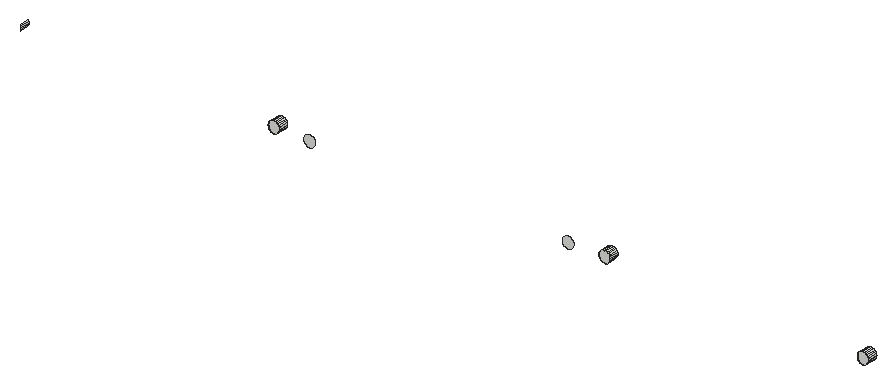
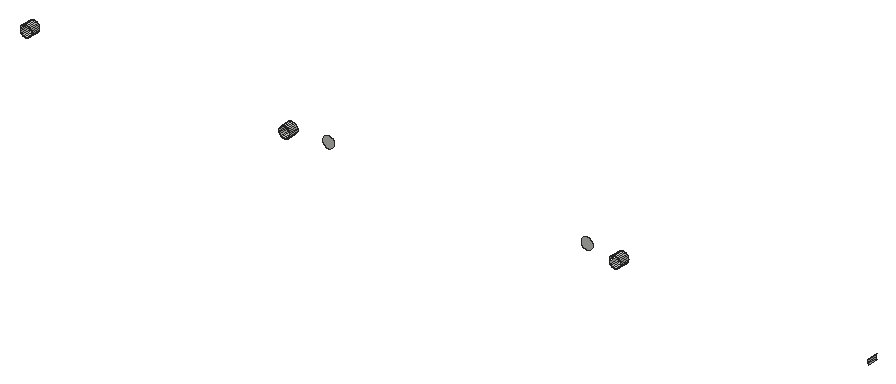
# SketchUp Ruby script. Lengths in inches.
U = 1.inch
M = Sketchup.active_model
def pt(a) = Geom::Point3d.new(a.map { |v| v * U })
def face(e, loops, mat)
  f = e.add_face(loops[0].map { |a| pt(a) })
  loops[1..].each { |l| e.add_face(l.map { |a| pt(a) }).erase! }
  f.material = f.back_material = mat if mat
  f
end
# faces: each face lists its corners as indices into pts; further lists are holes
def faces(e, pts, list, mat = nil) = list.each { |f| face(e, (f[0].is_a?(Array) ? f : [f]).map { |l| l.map { |i| pts[i] } }, mat) }
# xy, xz, yz: faces in a plane at the given z, y or x. An outline is a flat list of corners, or four numbers for a rectangle; further outlines are holes
def ring(l) = l.size == 4 ? [[l[0], l[1]], [l[2], l[1]], [l[2], l[3]], [l[0], l[3]]] : l.each_slice(2).to_a
def flat(e, list, mat, &to3) = list.each { |f| face(e, (f[0].is_a?(Array) ? f : [f]).map { |l| ring(l).map { |u, v| to3.(u, v) } }, mat) }
def xy(e, z, list, mat = nil) = flat(e, list, mat) { |x, y| [x, y, z] }
def xz(e, y, list, mat = nil) = flat(e, list, mat) { |x, z| [x, y, z] }
def yz(e, x, list, mat = nil) = flat(e, list, mat) { |y, z| [x, y, z] }
def lines(e, pts, list) = list.each { |a, b| e.add_line(pt(pts[a]), pt(pts[b])) }
# prism: a flat outline (further loops are holes) pulled along v
def prism(e, loops, v, mat = nil)
  f = face(e, loops, mat); d = Geom::Vector3d.new(v.map { |x| x * U })
  f.pushpull(f.normal.samedirection?(d) ? d.length : -d.length)
end
def box(e, o, s, mat = nil) = prism(e, [[o, [o[0] + s[0], o[1], o[2]], [o[0] + s[0], o[1] + s[1], o[2]], [o[0], o[1] + s[1], o[2]]]], [0, 0, s[2]], mat)
def at(x, y, z, deg = 0) = Geom::Transformation.translation(pt([x, y, z])) * Geom::Transformation.rotation(ORIGIN, Z_AXIS, deg.degrees)
def axes(o, x, y, z) = Geom::Transformation.new([*x, 0, *y, 0, *z, 0, *pt(o).to_a, 1])
def part(name) = M.definitions.add(name)
# library, detail: a bought-in or finely detailed component or shape, given as its bounding box
def library(name, o, s) = part(name).tap { |d| box(d.entities, o, s) }
def detail(e, o, s) = box(e.add_group.entities, o, s)
def put(e, d, t, mat = nil) = e.add_instance(d, t).tap { |i| i.material = mat if mat }
def group(e, t, mat = nil) = e.add_group.tap { |g| g.transformation = t; g.material = mat if mat }.entities
root = M.entities
xz(root,799.91,[[3602.55,131.88,3602.85,131.92,3603.12,132.03,3603.35,132.21,3603.53,132.44,3603.64,132.71,3603.68,133,3603.64,133.29,3603.53,133.57,3603.35,133.8,3603.12,133.98,3602.85,134.09,3602.55,134.13,3602.26,134.09,3601.99,133.98,3601.76,133.8,3601.58,133.57,3601.47,133.29,3601.43,133,3601.47,132.71,3601.58,132.44,3601.76,132.21,3601.99,132.03,3602.26,131.92],[3609.6,131.88,3609.9,131.92,3610.17,132.03,3610.4,132.21,3610.58,132.44,3610.69,132.71,3610.73,133,3610.69,133.29,3610.58,133.57,3610.4,133.8,3610.17,133.98,3609.9,134.09,3609.6,134.13,3609.3125,134.09,3609.04,133.98,3608.81,133.8,3608.63,133.57,3608.52,133.29,3608.48,133,3608.52,132.71,3608.63,132.44,3608.81,132.21,3609.04,132.03,3609.3125,131.92],[3660.73,131.88,3661.02,131.92,3661.29,132.03,3661.53,132.21,3661.7,132.44,3661.82,132.71,3661.85,133,3661.82,133.29,3661.7,133.57,3661.53,133.8,3661.29,133.98,3661.02,134.09,3660.73,134.13,3660.4375,134.09,3660.17,133.98,3659.93,133.8,3659.76,133.57,3659.64,133.29,3659.6,133,3659.64,132.71,3659.76,132.44,3659.93,132.21,3660.17,132.03,3660.4375,131.92],[3667.91,131.88,3668.2,131.92,3668.47,132.03,3668.7,132.21,3668.88,132.44,3668.99,132.71,3669.03,133,3668.99,133.29,3668.88,133.57,3668.7,133.8,3668.47,133.98,3668.2,134.09,3667.91,134.13,3667.61,134.09,3667.34,133.98,3667.11,133.8,3666.93,133.57,3666.82,133.29,3666.78,133,3666.82,132.71,3666.93,132.44,3667.11,132.21,3667.34,132.03,3667.61,131.92],[3719.03,131.88,3719.32,131.92,3719.59,132.03,3719.83,132.21,3720,132.44,3720.12,132.71,3720.16,133,3720.12,133.29,3720,133.57,3719.83,133.8,3719.59,133.98,3719.32,134.09,3719.03,134.13,3718.74,134.09,3718.47,133.98,3718.24,133.8,3718.06,133.57,3717.94,133.29,3717.91,133,3717.94,132.71,3718.06,132.44,3718.24,132.21,3718.47,132.03,3718.74,131.92]])
p = [[3601.99,801.78,132.03],[3602.26,801.78,131.92],[3602.26,799.91,131.92],[3601.99,799.91,132.03],[3602.55,801.78,131.88],[3602.55,799.91,131.88],
  [3602.85,801.78,131.92],[3602.85,799.91,131.92],[3603.12,801.78,132.03],[3603.12,799.91,132.03],[3667.34,801.78,132.03],[3667.61,801.78,131.92],
  [3667.61,799.91,131.92],[3667.34,799.91,132.03],[3667.91,801.78,131.88],[3667.91,799.91,131.88],[3668.2,801.78,131.92],[3668.2,799.91,131.92],
  [3668.47,801.78,132.03],[3668.47,799.91,132.03],[3718.47,801.78,132.03],[3718.74,801.78,131.92],[3718.74,799.91,131.92],[3718.47,799.91,132.03],
  [3719.03,801.78,131.88],[3719.03,799.91,131.88],[3719.32,801.78,131.92],[3719.32,799.91,131.92],[3719.59,801.78,132.03],[3719.59,799.91,132.03],
  [3601.76,801.78,132.21],[3601.76,799.91,132.21],[3603.35,801.78,132.21],[3603.35,799.91,132.21],[3667.11,801.78,132.21],[3667.11,799.91,132.21],
  [3668.7,801.78,132.21],[3668.7,799.91,132.21],[3718.24,801.78,132.21],[3718.24,799.91,132.21],[3719.83,801.78,132.21],[3719.83,799.91,132.21],
  [3601.58,801.78,132.44],[3601.58,799.91,132.44],[3603.53,801.78,132.44],[3603.53,799.91,132.44],[3666.93,801.78,132.44],[3666.93,799.91,132.44],
  [3668.88,801.78,132.44],[3668.88,799.91,132.44],[3718.06,801.78,132.44],[3718.06,799.91,132.44],[3720,801.78,132.44],[3720,799.91,132.44],
  [3552.4,801.78,132.44],[3552.52,801.78,132.71],[3552.52,799.91,132.71],[3552.4,799.91,132.44],[3601.47,801.78,132.71],[3601.47,799.91,132.71],
  [3603.64,801.78,132.71],[3603.64,799.91,132.71],[3666.82,801.78,132.71],[3666.82,799.91,132.71],[3668.99,801.78,132.71],[3668.99,799.91,132.71],
  [3717.94,801.78,132.71],[3717.94,799.91,132.71],[3720.12,801.78,132.71],[3720.12,799.91,132.71],[3552.55,801.78,133],[3552.55,799.91,133],
  [3601.43,801.78,133],[3601.43,799.91,133],[3666.78,801.78,133],[3666.78,799.91,133],[3669.03,801.78,133],[3669.03,799.91,133],
  [3717.91,801.78,133],[3717.91,799.91,133],[3720.16,801.78,133],[3720.16,799.91,133],[3552.52,801.78,133.29],[3552.52,799.91,133.29],
  [3601.47,801.78,133.29],[3601.47,799.91,133.29],[3603.68,801.78,133],[3603.64,801.78,133.29],[3603.64,799.91,133.29],[3603.68,799.91,133],
  [3666.82,801.78,133.29],[3666.82,799.91,133.29],[3668.99,801.78,133.29],[3668.99,799.91,133.29],[3717.94,801.78,133.29],[3717.94,799.91,133.29],
  [3720.12,801.78,133.29],[3720.12,799.91,133.29],[3552.4,801.78,133.57],[3552.4,799.91,133.57],[3601.58,801.78,133.57],[3601.58,799.91,133.57],
  [3603.53,801.78,133.57],[3603.53,799.91,133.57],[3666.93,801.78,133.57],[3666.93,799.91,133.57],[3668.88,801.78,133.57],[3668.88,799.91,133.57],
  [3718.06,801.78,133.57],[3718.06,799.91,133.57],[3720,801.78,133.57],[3720,799.91,133.57],[3601.76,801.78,133.8],[3601.76,799.91,133.8],
  [3603.35,801.78,133.8],[3603.35,799.91,133.8],[3667.11,801.78,133.8],[3667.11,799.91,133.8],[3668.7,801.78,133.8],[3668.7,799.91,133.8],
  [3718.24,801.78,133.8],[3718.24,799.91,133.8],[3719.83,801.78,133.8],[3719.83,799.91,133.8],[3601.99,801.78,133.98],[3601.99,799.91,133.98],
  [3603.12,801.78,133.98],[3603.12,799.91,133.98],[3667.34,801.78,133.98],[3667.34,799.91,133.98],[3668.47,801.78,133.98],[3668.47,799.91,133.98],
  [3718.47,801.78,133.98],[3718.47,799.91,133.98],[3719.59,801.78,133.98],[3719.59,799.91,133.98],[3602.26,801.78,134.09],[3602.26,799.91,134.09],
  [3602.85,801.78,134.09],[3602.85,799.91,134.09],[3667.61,801.78,134.09],[3667.61,799.91,134.09],[3668.2,801.78,134.09],[3668.2,799.91,134.09],
  [3718.74,801.78,134.09],[3718.74,799.91,134.09],[3719.32,801.78,134.09],[3719.32,799.91,134.09],[3602.55,801.78,134.13],[3602.55,799.91,134.13],
  [3667.91,801.78,134.13],[3667.91,799.91,134.13],[3719.03,801.78,134.13],[3719.03,799.91,134.13]]
faces(root,p,[[0,1,2,3],[1,4,5,2],[4,6,7,5],[6,8,9,7],[10,11,12,13],[11,14,15,12],[14,16,17,15],[16,18,19,17],
  [20,21,22,23],[21,24,25,22],[24,26,27,25],[26,28,29,27],[30,0,3,31],[8,32,33,9],[34,10,13,35],[18,36,37,19],
  [38,20,23,39],[28,40,41,29],[42,30,31,43],[32,44,45,33],[46,34,35,47],[36,48,49,37],[50,38,39,51],[40,52,53,41],
  [54,55,56,57],[58,42,43,59],[44,60,61,45],[62,46,47,63],[48,64,65,49],[66,50,51,67],[52,68,69,53],[55,70,71,56],
  [72,58,59,73],[74,62,63,75],[64,76,77,65],[78,66,67,79],[68,80,81,69],[70,82,83,71],[84,72,73,85],[86,87,88,89],
  [90,74,75,91],[76,92,93,77],[94,78,79,95],[80,96,97,81],[82,98,99,83],[100,84,85,101],[87,102,103,88],[104,90,91,105],
  [92,106,107,93],[108,94,95,109],[96,110,111,97],[112,100,101,113],[102,114,115,103],[116,104,105,117],[106,118,119,107],[120,108,109,121],
  [110,122,123,111],[124,112,113,125],[114,126,127,115],[128,116,117,129],[118,130,131,119],[132,120,121,133],[122,134,135,123],[136,124,125,137],
  [126,138,139,127],[140,128,129,141],[130,142,143,131],[144,132,133,145],[134,146,147,135],[148,136,137,149],[138,148,149,139],[150,140,141,151],
  [142,150,151,143],[152,144,145,153],[146,152,153,147]])
